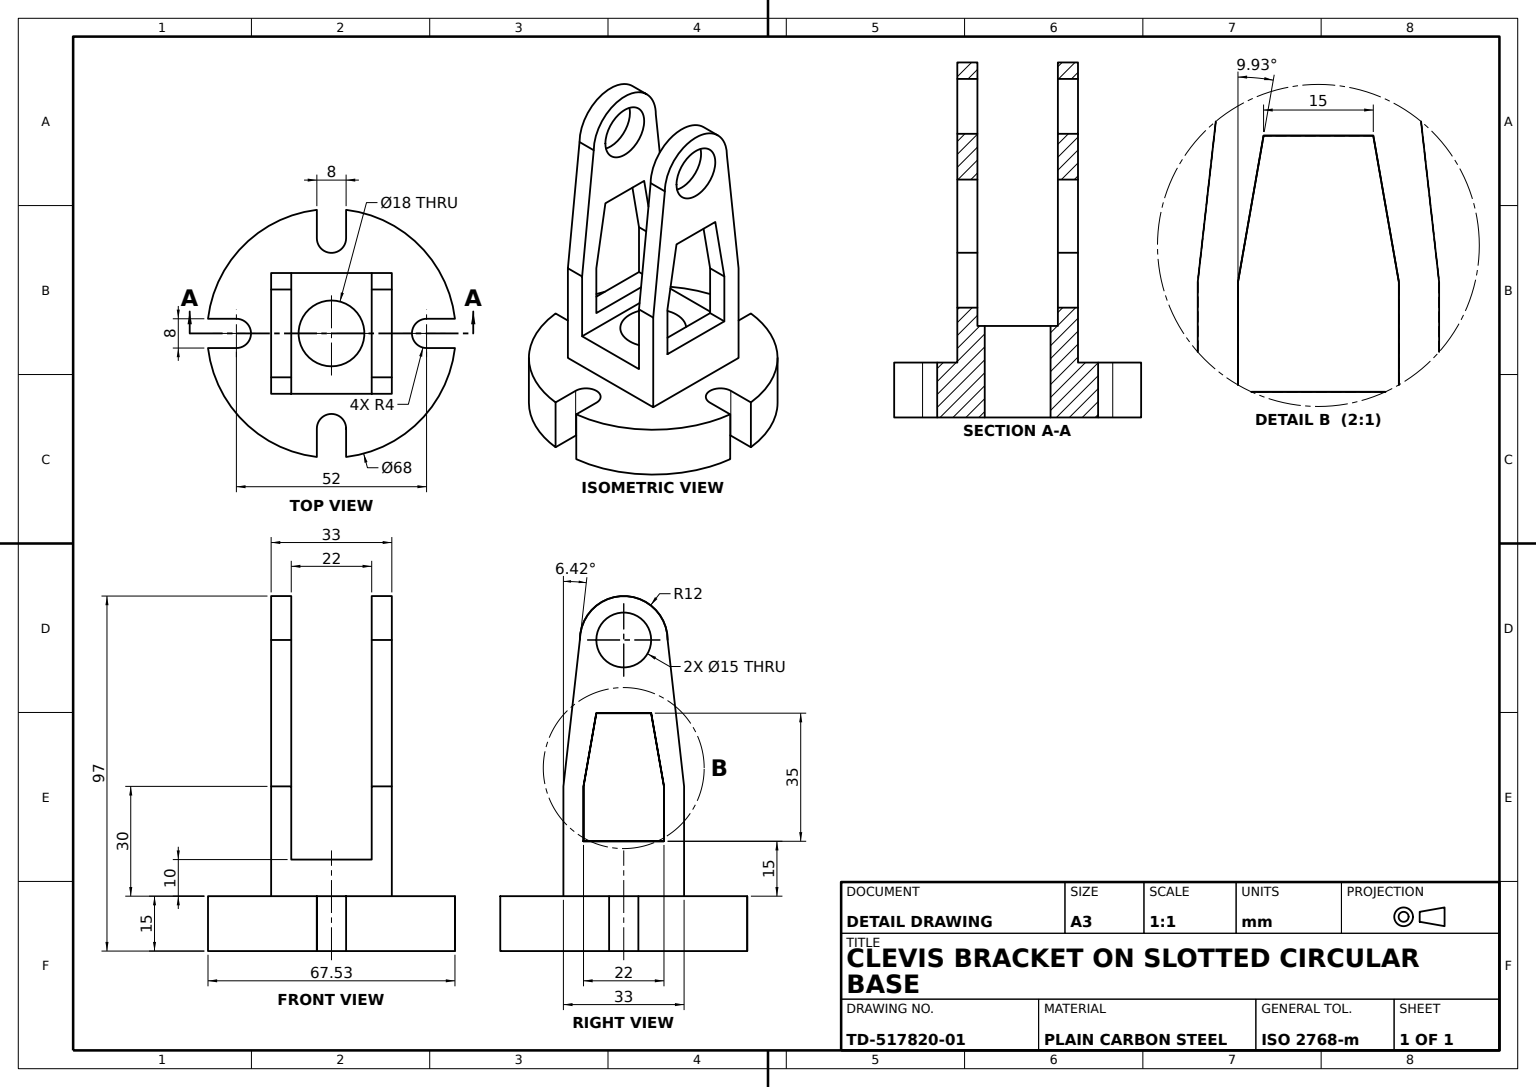
ISO-10303-21;
HEADER;
FILE_DESCRIPTION((''),'2;1');
FILE_NAME('','',(''),(''),'','','');
FILE_SCHEMA(('AUTOMOTIVE_DESIGN'));
ENDSEC;
DATA;
#1=APPLICATION_CONTEXT('');
#2=PRODUCT_CONTEXT('',#1,'mechanical');
#3=PRODUCT('','','',(#2));
#4=PRODUCT_DEFINITION_FORMATION('','',#3);
#5=PRODUCT_DEFINITION_CONTEXT('',#1,'design');
#6=PRODUCT_DEFINITION('','',#4,#5);
#7=PRODUCT_DEFINITION_SHAPE('','',#6);
#8=(LENGTH_UNIT()NAMED_UNIT(*)SI_UNIT(.MILLI.,.METRE.));
#9=(NAMED_UNIT(*)PLANE_ANGLE_UNIT()SI_UNIT($,.RADIAN.));
#10=(NAMED_UNIT(*)SI_UNIT($,.STERADIAN.)SOLID_ANGLE_UNIT());
#11=UNCERTAINTY_MEASURE_WITH_UNIT(LENGTH_MEASURE(1.E-05),#8,'distance_accuracy_value','');
#12=(GEOMETRIC_REPRESENTATION_CONTEXT(3)GLOBAL_UNCERTAINTY_ASSIGNED_CONTEXT((#11))GLOBAL_UNIT_ASSIGNED_CONTEXT((#8,#9,#10))REPRESENTATION_CONTEXT('',''));
#13=CARTESIAN_POINT('',(-33.763886,15.,-4.));
#14=VERTEX_POINT('',#13);
#15=CARTESIAN_POINT('',(-33.763886,0.,-4.));
#16=VERTEX_POINT('',#15);
#17=DIRECTION('',(0.,-1.,0.));
#18=VECTOR('',#17,1000.);
#19=LINE('',#13,#18);
#20=EDGE_CURVE('',#14,#16,#19,.T.);
#21=ORIENTED_EDGE('',*,*,#20,.F.);
#22=CARTESIAN_POINT('',(-4.,15.,-33.763886));
#23=VERTEX_POINT('',#22);
#24=CARTESIAN_POINT('',(0.,15.,0.));
#25=DIRECTION('',(0.,1.,0.));
#26=DIRECTION('',(0.,0.,1.));
#27=AXIS2_PLACEMENT_3D('',#24,#25,#26);
#28=CIRCLE('',#27,34.);
#29=EDGE_CURVE('',#23,#14,#28,.T.);
#30=ORIENTED_EDGE('',*,*,#29,.F.);
#31=CARTESIAN_POINT('',(-4.,0.,-33.763886));
#32=VERTEX_POINT('',#31);
#33=LINE('',#22,#18);
#34=EDGE_CURVE('',#23,#32,#33,.T.);
#35=ORIENTED_EDGE('',*,*,#34,.T.);
#36=CARTESIAN_POINT('',(0.,0.,0.));
#37=AXIS2_PLACEMENT_3D('',#36,#25,#26);
#38=CIRCLE('',#37,34.);
#39=EDGE_CURVE('',#32,#16,#38,.T.);
#40=ORIENTED_EDGE('',*,*,#39,.T.);
#41=EDGE_LOOP('',(#21,#30,#35,#40));
#42=FACE_OUTER_BOUND('',#41,.T.);
#43=DIRECTION('',(0.,0.,-1.));
#44=AXIS2_PLACEMENT_3D('',#24,#17,#43);
#45=CYLINDRICAL_SURFACE('',#44,34.);
#46=ADVANCED_FACE('',(#42),#45,.T.);
#47=CARTESIAN_POINT('',(11.,30.,11.));
#48=VERTEX_POINT('',#47);
#49=CARTESIAN_POINT('',(16.5,30.,11.));
#50=VERTEX_POINT('',#49);
#51=CARTESIAN_POINT('',(-37.5,30.,11.));
#52=DIRECTION('',(1.,0.,0.));
#53=VECTOR('',#52,1000.);
#54=LINE('',#51,#53);
#55=EDGE_CURVE('',#48,#50,#54,.T.);
#56=ORIENTED_EDGE('',*,*,#55,.T.);
#57=CARTESIAN_POINT('',(16.5,30.,-11.));
#58=VERTEX_POINT('',#57);
#59=CARTESIAN_POINT('',(16.5,30.,0.));
#60=VECTOR('',#43,1000.);
#61=LINE('',#59,#60);
#62=EDGE_CURVE('',#50,#58,#61,.T.);
#63=ORIENTED_EDGE('',*,*,#62,.T.);
#64=CARTESIAN_POINT('',(11.,30.,-11.));
#65=VERTEX_POINT('',#64);
#66=CARTESIAN_POINT('',(-37.5,30.,-11.));
#67=LINE('',#66,#53);
#68=EDGE_CURVE('',#65,#58,#67,.T.);
#69=ORIENTED_EDGE('',*,*,#68,.F.);
#70=CARTESIAN_POINT('',(11.,30.,0.));
#71=LINE('',#70,#60);
#72=EDGE_CURVE('',#48,#65,#71,.T.);
#73=ORIENTED_EDGE('',*,*,#72,.F.);
#74=EDGE_LOOP('',(#56,#63,#69,#73));
#75=FACE_OUTER_BOUND('',#74,.T.);
#76=CARTESIAN_POINT('',(-37.5,30.,0.));
#77=AXIS2_PLACEMENT_3D('',#76,#17,#43);
#78=PLANE('',#77);
#79=ADVANCED_FACE('',(#75),#78,.F.);
#80=CARTESIAN_POINT('',(4.,0.,26.));
#81=VERTEX_POINT('',#80);
#82=CARTESIAN_POINT('',(0.,0.,22.));
#83=VERTEX_POINT('',#82);
#84=CARTESIAN_POINT('',(0.,0.,26.));
#85=AXIS2_PLACEMENT_3D('',#84,#25,#26);
#86=CIRCLE('',#85,4.);
#87=EDGE_CURVE('',#81,#83,#86,.T.);
#88=ORIENTED_EDGE('',*,*,#87,.F.);
#89=CARTESIAN_POINT('',(4.,15.,26.));
#90=VERTEX_POINT('',#89);
#91=LINE('',#89,#18);
#92=EDGE_CURVE('',#90,#81,#91,.T.);
#93=ORIENTED_EDGE('',*,*,#92,.F.);
#94=CARTESIAN_POINT('',(0.,15.,22.));
#95=VERTEX_POINT('',#94);
#96=CARTESIAN_POINT('',(0.,15.,26.));
#97=AXIS2_PLACEMENT_3D('',#96,#25,#26);
#98=CIRCLE('',#97,4.);
#99=EDGE_CURVE('',#90,#95,#98,.T.);
#100=ORIENTED_EDGE('',*,*,#99,.T.);
#101=LINE('',#94,#18);
#102=EDGE_CURVE('',#95,#83,#101,.T.);
#103=ORIENTED_EDGE('',*,*,#102,.T.);
#104=EDGE_LOOP('',(#88,#93,#100,#103));
#105=FACE_OUTER_BOUND('',#104,.T.);
#106=AXIS2_PLACEMENT_3D('',#96,#17,#43);
#107=CYLINDRICAL_SURFACE('',#106,4.);
#108=ADVANCED_FACE('',(#105),#107,.F.);
#109=CARTESIAN_POINT('',(-11.,30.,11.));
#110=VERTEX_POINT('',#109);
#111=CARTESIAN_POINT('',(-11.,30.,-11.));
#112=VERTEX_POINT('',#111);
#113=CARTESIAN_POINT('',(-11.,30.,0.));
#114=LINE('',#113,#60);
#115=EDGE_CURVE('',#110,#112,#114,.T.);
#116=ORIENTED_EDGE('',*,*,#115,.T.);
#117=CARTESIAN_POINT('',(-16.5,30.,-11.));
#118=VERTEX_POINT('',#117);
#119=EDGE_CURVE('',#118,#112,#67,.T.);
#120=ORIENTED_EDGE('',*,*,#119,.F.);
#121=CARTESIAN_POINT('',(-16.5,30.,11.));
#122=VERTEX_POINT('',#121);
#123=CARTESIAN_POINT('',(-16.5,30.,0.));
#124=VECTOR('',#26,1000.);
#125=LINE('',#123,#124);
#126=EDGE_CURVE('',#118,#122,#125,.T.);
#127=ORIENTED_EDGE('',*,*,#126,.T.);
#128=EDGE_CURVE('',#122,#110,#54,.T.);
#129=ORIENTED_EDGE('',*,*,#128,.T.);
#130=EDGE_LOOP('',(#116,#120,#127,#129));
#131=FACE_OUTER_BOUND('',#130,.T.);
#132=ADVANCED_FACE('',(#131),#78,.F.);
#133=CARTESIAN_POINT('',(-16.5,15.,16.5));
#134=VERTEX_POINT('',#133);
#135=CARTESIAN_POINT('',(-16.5,15.,-16.5));
#136=VERTEX_POINT('',#135);
#137=CARTESIAN_POINT('',(-16.5,15.,0.));
#138=LINE('',#137,#60);
#139=EDGE_CURVE('',#134,#136,#138,.T.);
#140=ORIENTED_EDGE('',*,*,#139,.F.);
#141=CARTESIAN_POINT('',(-16.5,45.,16.5));
#142=VERTEX_POINT('',#141);
#143=CARTESIAN_POINT('',(-16.5,85.,16.5));
#144=LINE('',#143,#18);
#145=EDGE_CURVE('',#142,#134,#144,.T.);
#146=ORIENTED_EDGE('',*,*,#145,.F.);
#147=CARTESIAN_POINT('',(-16.5,85.,12.));
#148=VERTEX_POINT('',#147);
#149=CARTESIAN_POINT('',(-16.5,86.333128,11.850023));
#150=DIRECTION('',(0.,0.993731316,-0.111794773));
#151=VECTOR('',#150,1000.);
#152=LINE('',#149,#151);
#153=EDGE_CURVE('',#142,#148,#152,.T.);
#154=ORIENTED_EDGE('',*,*,#153,.T.);
#155=CARTESIAN_POINT('',(-16.5,85.,-12.));
#156=VERTEX_POINT('',#155);
#157=CARTESIAN_POINT('',(-16.5,85.,0.));
#158=DIRECTION('',(-1.,0.,0.));
#159=AXIS2_PLACEMENT_3D('',#157,#158,#26);
#160=CIRCLE('',#159,12.);
#161=EDGE_CURVE('',#148,#156,#160,.T.);
#162=ORIENTED_EDGE('',*,*,#161,.T.);
#163=CARTESIAN_POINT('',(-16.5,45.,-16.5));
#164=VERTEX_POINT('',#163);
#165=CARTESIAN_POINT('',(-16.5,86.333128,-11.850023));
#166=DIRECTION('',(0.,0.993731316,0.111794773));
#167=VECTOR('',#166,1000.);
#168=LINE('',#165,#167);
#169=EDGE_CURVE('',#164,#156,#168,.T.);
#170=ORIENTED_EDGE('',*,*,#169,.F.);
#171=CARTESIAN_POINT('',(-16.5,85.,-16.5));
#172=LINE('',#171,#18);
#173=EDGE_CURVE('',#164,#136,#172,.T.);
#174=ORIENTED_EDGE('',*,*,#173,.T.);
#175=EDGE_LOOP('',(#140,#146,#154,#162,#170,#174));
#176=FACE_OUTER_BOUND('',#175,.T.);
#177=CARTESIAN_POINT('',(-16.5,85.,-7.5));
#178=VERTEX_POINT('',#177);
#179=CARTESIAN_POINT('',(-16.5,85.,7.5));
#180=VERTEX_POINT('',#179);
#181=CIRCLE('',#159,7.5);
#182=EDGE_CURVE('',#178,#180,#181,.T.);
#183=ORIENTED_EDGE('',*,*,#182,.F.);
#184=EDGE_CURVE('',#180,#178,#181,.T.);
#185=ORIENTED_EDGE('',*,*,#184,.F.);
#186=EDGE_LOOP('',(#183,#185));
#187=FACE_BOUND('',#186,.T.);
#188=CARTESIAN_POINT('',(-16.5,45.,11.));
#189=VERTEX_POINT('',#188);
#190=CARTESIAN_POINT('',(-16.5,85.,11.));
#191=LINE('',#190,#18);
#192=EDGE_CURVE('',#189,#122,#191,.T.);
#193=ORIENTED_EDGE('',*,*,#192,.T.);
#194=ORIENTED_EDGE('',*,*,#126,.F.);
#195=CARTESIAN_POINT('',(-16.5,45.,-11.));
#196=VERTEX_POINT('',#195);
#197=CARTESIAN_POINT('',(-16.5,85.,-11.));
#198=LINE('',#197,#18);
#199=EDGE_CURVE('',#196,#118,#198,.T.);
#200=ORIENTED_EDGE('',*,*,#199,.F.);
#201=CARTESIAN_POINT('',(-16.5,65.,-7.5));
#202=VERTEX_POINT('',#201);
#203=CARTESIAN_POINT('',(-16.5,85.6792,-3.88114));
#204=DIRECTION('',(0.,0.985030467,0.172380332));
#205=VECTOR('',#204,1000.);
#206=LINE('',#203,#205);
#207=EDGE_CURVE('',#196,#202,#206,.T.);
#208=ORIENTED_EDGE('',*,*,#207,.T.);
#209=CARTESIAN_POINT('',(-16.5,65.,7.5));
#210=VERTEX_POINT('',#209);
#211=CARTESIAN_POINT('',(-16.5,65.,0.));
#212=LINE('',#211,#124);
#213=EDGE_CURVE('',#202,#210,#212,.T.);
#214=ORIENTED_EDGE('',*,*,#213,.T.);
#215=CARTESIAN_POINT('',(-16.5,85.6792,3.88114));
#216=DIRECTION('',(0.,0.985030467,-0.172380332));
#217=VECTOR('',#216,1000.);
#218=LINE('',#215,#217);
#219=EDGE_CURVE('',#189,#210,#218,.T.);
#220=ORIENTED_EDGE('',*,*,#219,.F.);
#221=EDGE_LOOP('',(#193,#194,#200,#208,#214,#220));
#222=FACE_BOUND('',#221,.T.);
#223=PLANE('',#159);
#224=ADVANCED_FACE('',(#176,#187,#222),#223,.T.);
#225=CARTESIAN_POINT('',(11.,85.,7.5));
#226=VERTEX_POINT('',#225);
#227=CARTESIAN_POINT('',(16.5,85.,7.5));
#228=VERTEX_POINT('',#227);
#229=CARTESIAN_POINT('',(-37.5,85.,7.5));
#230=LINE('',#229,#53);
#231=EDGE_CURVE('',#226,#228,#230,.T.);
#232=ORIENTED_EDGE('',*,*,#231,.T.);
#233=CARTESIAN_POINT('',(16.5,85.,-7.5));
#234=VERTEX_POINT('',#233);
#235=CARTESIAN_POINT('',(16.5,85.,0.));
#236=AXIS2_PLACEMENT_3D('',#235,#52,#43);
#237=CIRCLE('',#236,7.5);
#238=EDGE_CURVE('',#228,#234,#237,.T.);
#239=ORIENTED_EDGE('',*,*,#238,.T.);
#240=CARTESIAN_POINT('',(11.,85.,-7.5));
#241=VERTEX_POINT('',#240);
#242=CARTESIAN_POINT('',(-37.5,85.,-7.5));
#243=LINE('',#242,#53);
#244=EDGE_CURVE('',#241,#234,#243,.T.);
#245=ORIENTED_EDGE('',*,*,#244,.F.);
#246=CARTESIAN_POINT('',(11.,85.,0.));
#247=AXIS2_PLACEMENT_3D('',#246,#52,#43);
#248=CIRCLE('',#247,7.5);
#249=EDGE_CURVE('',#226,#241,#248,.T.);
#250=ORIENTED_EDGE('',*,*,#249,.F.);
#251=EDGE_LOOP('',(#232,#239,#245,#250));
#252=FACE_OUTER_BOUND('',#251,.T.);
#253=CARTESIAN_POINT('',(-37.5,85.,0.));
#254=AXIS2_PLACEMENT_3D('',#253,#52,#43);
#255=CYLINDRICAL_SURFACE('',#254,7.5);
#256=ADVANCED_FACE('',(#252),#255,.F.);
#257=CARTESIAN_POINT('',(11.,65.,7.5));
#258=VERTEX_POINT('',#257);
#259=CARTESIAN_POINT('',(11.,45.,11.));
#260=VERTEX_POINT('',#259);
#261=CARTESIAN_POINT('',(11.,85.6792,3.88114));
#262=DIRECTION('',(0.,-0.985030467,0.172380332));
#263=VECTOR('',#262,1000.);
#264=LINE('',#261,#263);
#265=EDGE_CURVE('',#258,#260,#264,.T.);
#266=ORIENTED_EDGE('',*,*,#265,.F.);
#267=CARTESIAN_POINT('',(16.5,65.,7.5));
#268=VERTEX_POINT('',#267);
#269=CARTESIAN_POINT('',(-37.5,65.,7.5));
#270=LINE('',#269,#53);
#271=EDGE_CURVE('',#258,#268,#270,.T.);
#272=ORIENTED_EDGE('',*,*,#271,.T.);
#273=CARTESIAN_POINT('',(16.5,45.,11.));
#274=VERTEX_POINT('',#273);
#275=CARTESIAN_POINT('',(16.5,3.204973,18.31413));
#276=LINE('',#275,#263);
#277=EDGE_CURVE('',#268,#274,#276,.T.);
#278=ORIENTED_EDGE('',*,*,#277,.T.);
#279=CARTESIAN_POINT('',(-37.5,45.,11.));
#280=LINE('',#279,#53);
#281=EDGE_CURVE('',#260,#274,#280,.T.);
#282=ORIENTED_EDGE('',*,*,#281,.F.);
#283=EDGE_LOOP('',(#266,#272,#278,#282));
#284=FACE_OUTER_BOUND('',#283,.T.);
#285=CARTESIAN_POINT('',(-37.5,3.204973,18.31413));
#286=DIRECTION('',(0.,0.172380332,0.985030467));
#287=AXIS2_PLACEMENT_3D('',#285,#286,#262);
#288=PLANE('',#287);
#289=ADVANCED_FACE('',(#284),#288,.F.);
#290=CARTESIAN_POINT('',(-11.,85.,-12.));
#291=VERTEX_POINT('',#290);
#292=CARTESIAN_POINT('',(-11.,45.,-16.5));
#293=VERTEX_POINT('',#292);
#294=CARTESIAN_POINT('',(-11.,86.333128,-11.850023));
#295=DIRECTION('',(0.,-0.993731316,-0.111794773));
#296=VECTOR('',#295,1000.);
#297=LINE('',#294,#296);
#298=EDGE_CURVE('',#291,#293,#297,.T.);
#299=ORIENTED_EDGE('',*,*,#298,.T.);
#300=CARTESIAN_POINT('',(-37.5,45.,-16.5));
#301=LINE('',#300,#53);
#302=EDGE_CURVE('',#164,#293,#301,.T.);
#303=ORIENTED_EDGE('',*,*,#302,.F.);
#304=ORIENTED_EDGE('',*,*,#169,.T.);
#305=CARTESIAN_POINT('',(0.,85.,-12.));
#306=LINE('',#305,#53);
#307=EDGE_CURVE('',#156,#291,#306,.T.);
#308=ORIENTED_EDGE('',*,*,#307,.T.);
#309=EDGE_LOOP('',(#299,#303,#304,#308));
#310=FACE_OUTER_BOUND('',#309,.T.);
#311=CARTESIAN_POINT('',(-37.5,2.395464,-21.29301));
#312=DIRECTION('',(0.,-0.111794773,0.993731316));
#313=AXIS2_PLACEMENT_3D('',#311,#312,#295);
#314=PLANE('',#313);
#315=ADVANCED_FACE('',(#310),#314,.F.);
#316=CARTESIAN_POINT('',(33.763886,15.,-4.));
#317=VERTEX_POINT('',#316);
#318=CARTESIAN_POINT('',(33.763886,0.,-4.));
#319=VERTEX_POINT('',#318);
#320=LINE('',#316,#18);
#321=EDGE_CURVE('',#317,#319,#320,.T.);
#322=ORIENTED_EDGE('',*,*,#321,.T.);
#323=CARTESIAN_POINT('',(4.,0.,-33.763886));
#324=VERTEX_POINT('',#323);
#325=EDGE_CURVE('',#319,#324,#38,.T.);
#326=ORIENTED_EDGE('',*,*,#325,.T.);
#327=CARTESIAN_POINT('',(4.,15.,-33.763886));
#328=VERTEX_POINT('',#327);
#329=LINE('',#327,#18);
#330=EDGE_CURVE('',#328,#324,#329,.T.);
#331=ORIENTED_EDGE('',*,*,#330,.F.);
#332=EDGE_CURVE('',#317,#328,#28,.T.);
#333=ORIENTED_EDGE('',*,*,#332,.F.);
#334=EDGE_LOOP('',(#322,#326,#331,#333));
#335=FACE_OUTER_BOUND('',#334,.T.);
#336=ADVANCED_FACE('',(#335),#45,.T.);
#337=CARTESIAN_POINT('',(0.,25.,-9.));
#338=VERTEX_POINT('',#337);
#339=CARTESIAN_POINT('',(0.,25.,9.));
#340=VERTEX_POINT('',#339);
#341=CARTESIAN_POINT('',(0.,25.,0.));
#342=AXIS2_PLACEMENT_3D('',#341,#17,#26);
#343=CIRCLE('',#342,9.);
#344=EDGE_CURVE('',#338,#340,#343,.T.);
#345=ORIENTED_EDGE('',*,*,#344,.T.);
#346=EDGE_CURVE('',#340,#338,#343,.T.);
#347=ORIENTED_EDGE('',*,*,#346,.T.);
#348=EDGE_LOOP('',(#345,#347));
#349=FACE_BOUND('',#348,.T.);
#350=CARTESIAN_POINT('',(11.,25.,-16.5));
#351=VERTEX_POINT('',#350);
#352=CARTESIAN_POINT('',(11.,25.,16.5));
#353=VERTEX_POINT('',#352);
#354=CARTESIAN_POINT('',(11.,25.,0.));
#355=LINE('',#354,#124);
#356=EDGE_CURVE('',#351,#353,#355,.T.);
#357=ORIENTED_EDGE('',*,*,#356,.F.);
#358=CARTESIAN_POINT('',(-11.,25.,-16.5));
#359=VERTEX_POINT('',#358);
#360=CARTESIAN_POINT('',(0.,25.,-16.5));
#361=LINE('',#360,#53);
#362=EDGE_CURVE('',#359,#351,#361,.T.);
#363=ORIENTED_EDGE('',*,*,#362,.F.);
#364=CARTESIAN_POINT('',(-11.,25.,16.5));
#365=VERTEX_POINT('',#364);
#366=CARTESIAN_POINT('',(-11.,25.,0.));
#367=LINE('',#366,#124);
#368=EDGE_CURVE('',#359,#365,#367,.T.);
#369=ORIENTED_EDGE('',*,*,#368,.T.);
#370=CARTESIAN_POINT('',(0.,25.,16.5));
#371=LINE('',#370,#53);
#372=EDGE_CURVE('',#365,#353,#371,.T.);
#373=ORIENTED_EDGE('',*,*,#372,.T.);
#374=EDGE_LOOP('',(#357,#363,#369,#373));
#375=FACE_OUTER_BOUND('',#374,.T.);
#376=AXIS2_PLACEMENT_3D('',#341,#25,#26);
#377=PLANE('',#376);
#378=ADVANCED_FACE('',(#349,#375),#377,.T.);
#379=CARTESIAN_POINT('',(-4.,15.,26.));
#380=VERTEX_POINT('',#379);
#381=CARTESIAN_POINT('',(-4.,0.,26.));
#382=VERTEX_POINT('',#381);
#383=LINE('',#379,#18);
#384=EDGE_CURVE('',#380,#382,#383,.T.);
#385=ORIENTED_EDGE('',*,*,#384,.T.);
#386=EDGE_CURVE('',#83,#382,#86,.T.);
#387=ORIENTED_EDGE('',*,*,#386,.F.);
#388=ORIENTED_EDGE('',*,*,#102,.F.);
#389=EDGE_CURVE('',#95,#380,#98,.T.);
#390=ORIENTED_EDGE('',*,*,#389,.T.);
#391=EDGE_LOOP('',(#385,#387,#388,#390));
#392=FACE_OUTER_BOUND('',#391,.T.);
#393=ADVANCED_FACE('',(#392),#107,.F.);
#394=CARTESIAN_POINT('',(-33.763886,15.,4.));
#395=VERTEX_POINT('',#394);
#396=CARTESIAN_POINT('',(-4.,15.,33.763886));
#397=VERTEX_POINT('',#396);
#398=EDGE_CURVE('',#395,#397,#28,.T.);
#399=ORIENTED_EDGE('',*,*,#398,.F.);
#400=CARTESIAN_POINT('',(-33.763886,0.,4.));
#401=VERTEX_POINT('',#400);
#402=LINE('',#394,#18);
#403=EDGE_CURVE('',#395,#401,#402,.T.);
#404=ORIENTED_EDGE('',*,*,#403,.T.);
#405=CARTESIAN_POINT('',(-4.,0.,33.763886));
#406=VERTEX_POINT('',#405);
#407=EDGE_CURVE('',#401,#406,#38,.T.);
#408=ORIENTED_EDGE('',*,*,#407,.T.);
#409=LINE('',#396,#18);
#410=EDGE_CURVE('',#397,#406,#409,.T.);
#411=ORIENTED_EDGE('',*,*,#410,.F.);
#412=EDGE_LOOP('',(#399,#404,#408,#411));
#413=FACE_OUTER_BOUND('',#412,.T.);
#414=ADVANCED_FACE('',(#413),#45,.T.);
#415=CARTESIAN_POINT('',(-11.,65.,7.5));
#416=VERTEX_POINT('',#415);
#417=EDGE_CURVE('',#210,#416,#270,.T.);
#418=ORIENTED_EDGE('',*,*,#417,.T.);
#419=CARTESIAN_POINT('',(-11.,45.,11.));
#420=VERTEX_POINT('',#419);
#421=CARTESIAN_POINT('',(-11.,85.6792,3.88114));
#422=LINE('',#421,#263);
#423=EDGE_CURVE('',#416,#420,#422,.T.);
#424=ORIENTED_EDGE('',*,*,#423,.T.);
#425=EDGE_CURVE('',#189,#420,#280,.T.);
#426=ORIENTED_EDGE('',*,*,#425,.F.);
#427=ORIENTED_EDGE('',*,*,#219,.T.);
#428=EDGE_LOOP('',(#418,#424,#426,#427));
#429=FACE_OUTER_BOUND('',#428,.T.);
#430=ADVANCED_FACE('',(#429),#288,.F.);
#431=CARTESIAN_POINT('',(11.,85.,-12.));
#432=VERTEX_POINT('',#431);
#433=CARTESIAN_POINT('',(11.,45.,-16.5));
#434=VERTEX_POINT('',#433);
#435=CARTESIAN_POINT('',(11.,86.333128,-11.850023));
#436=LINE('',#435,#296);
#437=EDGE_CURVE('',#432,#434,#436,.T.);
#438=ORIENTED_EDGE('',*,*,#437,.F.);
#439=CARTESIAN_POINT('',(16.5,85.,-12.));
#440=VERTEX_POINT('',#439);
#441=CARTESIAN_POINT('',(-37.5,85.,-12.));
#442=LINE('',#441,#53);
#443=EDGE_CURVE('',#432,#440,#442,.T.);
#444=ORIENTED_EDGE('',*,*,#443,.T.);
#445=CARTESIAN_POINT('',(16.5,45.,-16.5));
#446=VERTEX_POINT('',#445);
#447=CARTESIAN_POINT('',(16.5,2.395464,-21.29301));
#448=LINE('',#447,#296);
#449=EDGE_CURVE('',#440,#446,#448,.T.);
#450=ORIENTED_EDGE('',*,*,#449,.T.);
#451=EDGE_CURVE('',#434,#446,#301,.T.);
#452=ORIENTED_EDGE('',*,*,#451,.F.);
#453=EDGE_LOOP('',(#438,#444,#450,#452));
#454=FACE_OUTER_BOUND('',#453,.T.);
#455=ADVANCED_FACE('',(#454),#314,.F.);
#456=CARTESIAN_POINT('',(33.763886,15.,4.));
#457=VERTEX_POINT('',#456);
#458=CARTESIAN_POINT('',(33.763886,0.,4.));
#459=VERTEX_POINT('',#458);
#460=LINE('',#456,#18);
#461=EDGE_CURVE('',#457,#459,#460,.T.);
#462=ORIENTED_EDGE('',*,*,#461,.F.);
#463=CARTESIAN_POINT('',(4.,15.,33.763886));
#464=VERTEX_POINT('',#463);
#465=EDGE_CURVE('',#464,#457,#28,.T.);
#466=ORIENTED_EDGE('',*,*,#465,.F.);
#467=CARTESIAN_POINT('',(4.,0.,33.763886));
#468=VERTEX_POINT('',#467);
#469=LINE('',#463,#18);
#470=EDGE_CURVE('',#464,#468,#469,.T.);
#471=ORIENTED_EDGE('',*,*,#470,.T.);
#472=EDGE_CURVE('',#468,#459,#38,.T.);
#473=ORIENTED_EDGE('',*,*,#472,.T.);
#474=EDGE_LOOP('',(#462,#466,#471,#473));
#475=FACE_OUTER_BOUND('',#474,.T.);
#476=ADVANCED_FACE('',(#475),#45,.T.);
#477=ORIENTED_EDGE('',*,*,#470,.F.);
#478=CARTESIAN_POINT('',(4.,15.,0.));
#479=LINE('',#478,#124);
#480=EDGE_CURVE('',#90,#464,#479,.T.);
#481=ORIENTED_EDGE('',*,*,#480,.F.);
#482=ORIENTED_EDGE('',*,*,#92,.T.);
#483=CARTESIAN_POINT('',(4.,0.,0.));
#484=LINE('',#483,#124);
#485=EDGE_CURVE('',#81,#468,#484,.T.);
#486=ORIENTED_EDGE('',*,*,#485,.T.);
#487=EDGE_LOOP('',(#477,#481,#482,#486));
#488=FACE_OUTER_BOUND('',#487,.T.);
#489=AXIS2_PLACEMENT_3D('',#478,#52,#43);
#490=PLANE('',#489);
#491=ADVANCED_FACE('',(#488),#490,.F.);
#492=CARTESIAN_POINT('',(16.5,65.,-7.5));
#493=VERTEX_POINT('',#492);
#494=CARTESIAN_POINT('',(16.5,65.,0.));
#495=LINE('',#494,#60);
#496=EDGE_CURVE('',#268,#493,#495,.T.);
#497=ORIENTED_EDGE('',*,*,#496,.F.);
#498=ORIENTED_EDGE('',*,*,#271,.F.);
#499=CARTESIAN_POINT('',(11.,65.,-7.5));
#500=VERTEX_POINT('',#499);
#501=CARTESIAN_POINT('',(11.,65.,0.));
#502=LINE('',#501,#60);
#503=EDGE_CURVE('',#258,#500,#502,.T.);
#504=ORIENTED_EDGE('',*,*,#503,.T.);
#505=CARTESIAN_POINT('',(-37.5,65.,-7.5));
#506=LINE('',#505,#53);
#507=EDGE_CURVE('',#500,#493,#506,.T.);
#508=ORIENTED_EDGE('',*,*,#507,.T.);
#509=EDGE_LOOP('',(#497,#498,#504,#508));
#510=FACE_OUTER_BOUND('',#509,.T.);
#511=CARTESIAN_POINT('',(-37.5,65.,0.));
#512=AXIS2_PLACEMENT_3D('',#511,#17,#43);
#513=PLANE('',#512);
#514=ADVANCED_FACE('',(#510),#513,.T.);
#515=CARTESIAN_POINT('',(11.,45.,-11.));
#516=VERTEX_POINT('',#515);
#517=CARTESIAN_POINT('',(11.,85.6792,-3.88114));
#518=DIRECTION('',(0.,-0.985030467,-0.172380332));
#519=VECTOR('',#518,1000.);
#520=LINE('',#517,#519);
#521=EDGE_CURVE('',#500,#516,#520,.T.);
#522=ORIENTED_EDGE('',*,*,#521,.T.);
#523=CARTESIAN_POINT('',(16.5,45.,-11.));
#524=VERTEX_POINT('',#523);
#525=CARTESIAN_POINT('',(-37.5,45.,-11.));
#526=LINE('',#525,#53);
#527=EDGE_CURVE('',#516,#524,#526,.T.);
#528=ORIENTED_EDGE('',*,*,#527,.T.);
#529=CARTESIAN_POINT('',(16.5,3.204973,-18.31413));
#530=LINE('',#529,#519);
#531=EDGE_CURVE('',#493,#524,#530,.T.);
#532=ORIENTED_EDGE('',*,*,#531,.F.);
#533=ORIENTED_EDGE('',*,*,#507,.F.);
#534=EDGE_LOOP('',(#522,#528,#532,#533));
#535=FACE_OUTER_BOUND('',#534,.T.);
#536=CARTESIAN_POINT('',(-37.5,3.204973,-18.31413));
#537=DIRECTION('',(0.,-0.172380332,0.985030467));
#538=AXIS2_PLACEMENT_3D('',#536,#537,#518);
#539=PLANE('',#538);
#540=ADVANCED_FACE('',(#535),#539,.T.);
#541=EDGE_CURVE('',#234,#228,#237,.T.);
#542=ORIENTED_EDGE('',*,*,#541,.T.);
#543=ORIENTED_EDGE('',*,*,#231,.F.);
#544=EDGE_CURVE('',#241,#226,#248,.T.);
#545=ORIENTED_EDGE('',*,*,#544,.F.);
#546=ORIENTED_EDGE('',*,*,#244,.T.);
#547=EDGE_LOOP('',(#542,#543,#545,#546));
#548=FACE_OUTER_BOUND('',#547,.T.);
#549=ADVANCED_FACE('',(#548),#255,.F.);
#550=CARTESIAN_POINT('',(-4.,15.,-26.));
#551=VERTEX_POINT('',#550);
#552=CARTESIAN_POINT('',(-4.,0.,-26.));
#553=VERTEX_POINT('',#552);
#554=LINE('',#550,#18);
#555=EDGE_CURVE('',#551,#553,#554,.T.);
#556=ORIENTED_EDGE('',*,*,#555,.T.);
#557=CARTESIAN_POINT('',(-4.,0.,0.));
#558=LINE('',#557,#60);
#559=EDGE_CURVE('',#553,#32,#558,.T.);
#560=ORIENTED_EDGE('',*,*,#559,.T.);
#561=ORIENTED_EDGE('',*,*,#34,.F.);
#562=CARTESIAN_POINT('',(-4.,15.,0.));
#563=LINE('',#562,#60);
#564=EDGE_CURVE('',#551,#23,#563,.T.);
#565=ORIENTED_EDGE('',*,*,#564,.F.);
#566=EDGE_LOOP('',(#556,#560,#561,#565));
#567=FACE_OUTER_BOUND('',#566,.T.);
#568=AXIS2_PLACEMENT_3D('',#562,#158,#26);
#569=PLANE('',#568);
#570=ADVANCED_FACE('',(#567),#569,.F.);
#571=CARTESIAN_POINT('',(11.,45.,16.5));
#572=VERTEX_POINT('',#571);
#573=CARTESIAN_POINT('',(16.5,45.,16.5));
#574=VERTEX_POINT('',#573);
#575=CARTESIAN_POINT('',(-37.5,45.,16.5));
#576=LINE('',#575,#53);
#577=EDGE_CURVE('',#572,#574,#576,.T.);
#578=ORIENTED_EDGE('',*,*,#577,.T.);
#579=CARTESIAN_POINT('',(16.5,85.,12.));
#580=VERTEX_POINT('',#579);
#581=CARTESIAN_POINT('',(16.5,2.395464,21.29301));
#582=DIRECTION('',(0.,-0.993731316,0.111794773));
#583=VECTOR('',#582,1000.);
#584=LINE('',#581,#583);
#585=EDGE_CURVE('',#580,#574,#584,.T.);
#586=ORIENTED_EDGE('',*,*,#585,.F.);
#587=CARTESIAN_POINT('',(11.,85.,12.));
#588=VERTEX_POINT('',#587);
#589=CARTESIAN_POINT('',(-37.5,85.,12.));
#590=LINE('',#589,#53);
#591=EDGE_CURVE('',#588,#580,#590,.T.);
#592=ORIENTED_EDGE('',*,*,#591,.F.);
#593=CARTESIAN_POINT('',(11.,86.333128,11.850023));
#594=LINE('',#593,#583);
#595=EDGE_CURVE('',#588,#572,#594,.T.);
#596=ORIENTED_EDGE('',*,*,#595,.T.);
#597=EDGE_LOOP('',(#578,#586,#592,#596));
#598=FACE_OUTER_BOUND('',#597,.T.);
#599=CARTESIAN_POINT('',(-37.5,2.395464,21.29301));
#600=DIRECTION('',(0.,0.111794773,0.993731316));
#601=AXIS2_PLACEMENT_3D('',#599,#600,#582);
#602=PLANE('',#601);
#603=ADVANCED_FACE('',(#598),#602,.T.);
#604=CARTESIAN_POINT('',(-11.,85.,12.));
#605=VERTEX_POINT('',#604);
#606=CARTESIAN_POINT('',(0.,85.,12.));
#607=LINE('',#606,#53);
#608=EDGE_CURVE('',#148,#605,#607,.T.);
#609=ORIENTED_EDGE('',*,*,#608,.F.);
#610=ORIENTED_EDGE('',*,*,#153,.F.);
#611=CARTESIAN_POINT('',(-11.,45.,16.5));
#612=VERTEX_POINT('',#611);
#613=EDGE_CURVE('',#142,#612,#576,.T.);
#614=ORIENTED_EDGE('',*,*,#613,.T.);
#615=CARTESIAN_POINT('',(-11.,86.333128,11.850023));
#616=LINE('',#615,#583);
#617=EDGE_CURVE('',#605,#612,#616,.T.);
#618=ORIENTED_EDGE('',*,*,#617,.F.);
#619=EDGE_LOOP('',(#609,#610,#614,#618));
#620=FACE_OUTER_BOUND('',#619,.T.);
#621=ADVANCED_FACE('',(#620),#602,.T.);
#622=CARTESIAN_POINT('',(-11.,65.,-7.5));
#623=VERTEX_POINT('',#622);
#624=EDGE_CURVE('',#202,#623,#506,.T.);
#625=ORIENTED_EDGE('',*,*,#624,.T.);
#626=CARTESIAN_POINT('',(-11.,65.,0.));
#627=LINE('',#626,#60);
#628=EDGE_CURVE('',#416,#623,#627,.T.);
#629=ORIENTED_EDGE('',*,*,#628,.F.);
#630=ORIENTED_EDGE('',*,*,#417,.F.);
#631=ORIENTED_EDGE('',*,*,#213,.F.);
#632=EDGE_LOOP('',(#625,#629,#630,#631));
#633=FACE_OUTER_BOUND('',#632,.T.);
#634=ADVANCED_FACE('',(#633),#513,.T.);
#635=CARTESIAN_POINT('',(16.5,15.,16.5));
#636=VERTEX_POINT('',#635);
#637=CARTESIAN_POINT('',(16.5,85.,16.5));
#638=LINE('',#637,#18);
#639=EDGE_CURVE('',#574,#636,#638,.T.);
#640=ORIENTED_EDGE('',*,*,#639,.T.);
#641=CARTESIAN_POINT('',(16.5,15.,-16.5));
#642=VERTEX_POINT('',#641);
#643=CARTESIAN_POINT('',(16.5,15.,0.));
#644=LINE('',#643,#60);
#645=EDGE_CURVE('',#636,#642,#644,.T.);
#646=ORIENTED_EDGE('',*,*,#645,.T.);
#647=CARTESIAN_POINT('',(16.5,85.,-16.5));
#648=LINE('',#647,#18);
#649=EDGE_CURVE('',#446,#642,#648,.T.);
#650=ORIENTED_EDGE('',*,*,#649,.F.);
#651=ORIENTED_EDGE('',*,*,#449,.F.);
#652=CIRCLE('',#236,12.);
#653=EDGE_CURVE('',#440,#580,#652,.T.);
#654=ORIENTED_EDGE('',*,*,#653,.T.);
#655=ORIENTED_EDGE('',*,*,#585,.T.);
#656=EDGE_LOOP('',(#640,#646,#650,#651,#654,#655));
#657=FACE_OUTER_BOUND('',#656,.T.);
#658=CARTESIAN_POINT('',(16.5,0.,11.));
#659=VECTOR('',#25,1000.);
#660=LINE('',#658,#659);
#661=EDGE_CURVE('',#50,#274,#660,.T.);
#662=ORIENTED_EDGE('',*,*,#661,.T.);
#663=ORIENTED_EDGE('',*,*,#277,.F.);
#664=ORIENTED_EDGE('',*,*,#496,.T.);
#665=ORIENTED_EDGE('',*,*,#531,.T.);
#666=CARTESIAN_POINT('',(16.5,0.,-11.));
#667=LINE('',#666,#659);
#668=EDGE_CURVE('',#58,#524,#667,.T.);
#669=ORIENTED_EDGE('',*,*,#668,.F.);
#670=ORIENTED_EDGE('',*,*,#62,.F.);
#671=EDGE_LOOP('',(#662,#663,#664,#665,#669,#670));
#672=FACE_BOUND('',#671,.T.);
#673=ORIENTED_EDGE('',*,*,#238,.F.);
#674=ORIENTED_EDGE('',*,*,#541,.F.);
#675=EDGE_LOOP('',(#673,#674));
#676=FACE_BOUND('',#675,.T.);
#677=AXIS2_PLACEMENT_3D('',#235,#158,#26);
#678=PLANE('',#677);
#679=ADVANCED_FACE('',(#657,#672,#676),#678,.F.);
#680=ORIENTED_EDGE('',*,*,#20,.T.);
#681=CARTESIAN_POINT('',(-26.,0.,-4.));
#682=VERTEX_POINT('',#681);
#683=CARTESIAN_POINT('',(0.,0.,-4.));
#684=VECTOR('',#158,1000.);
#685=LINE('',#683,#684);
#686=EDGE_CURVE('',#682,#16,#685,.T.);
#687=ORIENTED_EDGE('',*,*,#686,.F.);
#688=CARTESIAN_POINT('',(-26.,15.,-4.));
#689=VERTEX_POINT('',#688);
#690=LINE('',#688,#18);
#691=EDGE_CURVE('',#689,#682,#690,.T.);
#692=ORIENTED_EDGE('',*,*,#691,.F.);
#693=CARTESIAN_POINT('',(0.,15.,-4.));
#694=LINE('',#693,#684);
#695=EDGE_CURVE('',#689,#14,#694,.T.);
#696=ORIENTED_EDGE('',*,*,#695,.T.);
#697=EDGE_LOOP('',(#680,#687,#692,#696));
#698=FACE_OUTER_BOUND('',#697,.T.);
#699=AXIS2_PLACEMENT_3D('',#693,#26,#52);
#700=PLANE('',#699);
#701=ADVANCED_FACE('',(#698),#700,.T.);
#702=ORIENTED_EDGE('',*,*,#281,.T.);
#703=ORIENTED_EDGE('',*,*,#661,.F.);
#704=ORIENTED_EDGE('',*,*,#55,.F.);
#705=CARTESIAN_POINT('',(11.,85.,11.));
#706=LINE('',#705,#659);
#707=EDGE_CURVE('',#48,#260,#706,.T.);
#708=ORIENTED_EDGE('',*,*,#707,.T.);
#709=EDGE_LOOP('',(#702,#703,#704,#708));
#710=FACE_OUTER_BOUND('',#709,.T.);
#711=CARTESIAN_POINT('',(-37.5,0.,11.));
#712=AXIS2_PLACEMENT_3D('',#711,#43,#25);
#713=PLANE('',#712);
#714=ADVANCED_FACE('',(#710),#713,.T.);
#715=ORIENTED_EDGE('',*,*,#544,.T.);
#716=ORIENTED_EDGE('',*,*,#249,.T.);
#717=EDGE_LOOP('',(#715,#716));
#718=FACE_BOUND('',#717,.T.);
#719=ORIENTED_EDGE('',*,*,#503,.F.);
#720=ORIENTED_EDGE('',*,*,#265,.T.);
#721=ORIENTED_EDGE('',*,*,#707,.F.);
#722=ORIENTED_EDGE('',*,*,#72,.T.);
#723=CARTESIAN_POINT('',(11.,85.,-11.));
#724=LINE('',#723,#659);
#725=EDGE_CURVE('',#65,#516,#724,.T.);
#726=ORIENTED_EDGE('',*,*,#725,.T.);
#727=ORIENTED_EDGE('',*,*,#521,.F.);
#728=EDGE_LOOP('',(#719,#720,#721,#722,#726,#727));
#729=FACE_BOUND('',#728,.T.);
#730=CARTESIAN_POINT('',(11.,85.,-16.5));
#731=LINE('',#730,#18);
#732=EDGE_CURVE('',#434,#351,#731,.T.);
#733=ORIENTED_EDGE('',*,*,#732,.T.);
#734=ORIENTED_EDGE('',*,*,#356,.T.);
#735=CARTESIAN_POINT('',(11.,85.,16.5));
#736=LINE('',#735,#18);
#737=EDGE_CURVE('',#572,#353,#736,.T.);
#738=ORIENTED_EDGE('',*,*,#737,.F.);
#739=ORIENTED_EDGE('',*,*,#595,.F.);
#740=CIRCLE('',#247,12.);
#741=EDGE_CURVE('',#432,#588,#740,.T.);
#742=ORIENTED_EDGE('',*,*,#741,.F.);
#743=ORIENTED_EDGE('',*,*,#437,.T.);
#744=EDGE_LOOP('',(#733,#734,#738,#739,#742,#743));
#745=FACE_OUTER_BOUND('',#744,.T.);
#746=PLANE('',#247);
#747=ADVANCED_FACE('',(#718,#729,#745),#746,.F.);
#748=CARTESIAN_POINT('',(0.,0.,-9.));
#749=VERTEX_POINT('',#748);
#750=LINE('',#748,#659);
#751=EDGE_CURVE('',#749,#338,#750,.T.);
#752=ORIENTED_EDGE('',*,*,#751,.F.);
#753=CARTESIAN_POINT('',(0.,0.,9.));
#754=VERTEX_POINT('',#753);
#755=CIRCLE('',#37,9.);
#756=EDGE_CURVE('',#754,#749,#755,.T.);
#757=ORIENTED_EDGE('',*,*,#756,.F.);
#758=LINE('',#753,#659);
#759=EDGE_CURVE('',#754,#340,#758,.T.);
#760=ORIENTED_EDGE('',*,*,#759,.T.);
#761=ORIENTED_EDGE('',*,*,#344,.F.);
#762=EDGE_LOOP('',(#752,#757,#760,#761));
#763=FACE_OUTER_BOUND('',#762,.T.);
#764=CYLINDRICAL_SURFACE('',#37,9.);
#765=ADVANCED_FACE('',(#763),#764,.F.);
#766=CARTESIAN_POINT('',(-11.,85.,7.5));
#767=VERTEX_POINT('',#766);
#768=CARTESIAN_POINT('',(-11.,85.,-7.5));
#769=VERTEX_POINT('',#768);
#770=CARTESIAN_POINT('',(-11.,85.,0.));
#771=AXIS2_PLACEMENT_3D('',#770,#52,#43);
#772=CIRCLE('',#771,7.5);
#773=EDGE_CURVE('',#767,#769,#772,.T.);
#774=ORIENTED_EDGE('',*,*,#773,.T.);
#775=EDGE_CURVE('',#178,#769,#243,.T.);
#776=ORIENTED_EDGE('',*,*,#775,.F.);
#777=ORIENTED_EDGE('',*,*,#182,.T.);
#778=EDGE_CURVE('',#180,#767,#230,.T.);
#779=ORIENTED_EDGE('',*,*,#778,.T.);
#780=EDGE_LOOP('',(#774,#776,#777,#779));
#781=FACE_OUTER_BOUND('',#780,.T.);
#782=ADVANCED_FACE('',(#781),#255,.F.);
#783=ORIENTED_EDGE('',*,*,#384,.F.);
#784=LINE('',#562,#124);
#785=EDGE_CURVE('',#380,#397,#784,.T.);
#786=ORIENTED_EDGE('',*,*,#785,.T.);
#787=ORIENTED_EDGE('',*,*,#410,.T.);
#788=LINE('',#557,#124);
#789=EDGE_CURVE('',#382,#406,#788,.T.);
#790=ORIENTED_EDGE('',*,*,#789,.F.);
#791=EDGE_LOOP('',(#783,#786,#787,#790));
#792=FACE_OUTER_BOUND('',#791,.T.);
#793=AXIS2_PLACEMENT_3D('',#562,#52,#43);
#794=PLANE('',#793);
#795=ADVANCED_FACE('',(#792),#794,.T.);
#796=CARTESIAN_POINT('',(-11.,45.,-11.));
#797=VERTEX_POINT('',#796);
#798=CARTESIAN_POINT('',(-11.,85.6792,-3.88114));
#799=LINE('',#798,#519);
#800=EDGE_CURVE('',#623,#797,#799,.T.);
#801=ORIENTED_EDGE('',*,*,#800,.F.);
#802=ORIENTED_EDGE('',*,*,#624,.F.);
#803=ORIENTED_EDGE('',*,*,#207,.F.);
#804=EDGE_CURVE('',#196,#797,#526,.T.);
#805=ORIENTED_EDGE('',*,*,#804,.T.);
#806=EDGE_LOOP('',(#801,#802,#803,#805));
#807=FACE_OUTER_BOUND('',#806,.T.);
#808=ADVANCED_FACE('',(#807),#539,.T.);
#809=ORIENTED_EDGE('',*,*,#737,.T.);
#810=ORIENTED_EDGE('',*,*,#372,.F.);
#811=CARTESIAN_POINT('',(-11.,85.,16.5));
#812=LINE('',#811,#18);
#813=EDGE_CURVE('',#612,#365,#812,.T.);
#814=ORIENTED_EDGE('',*,*,#813,.F.);
#815=ORIENTED_EDGE('',*,*,#613,.F.);
#816=ORIENTED_EDGE('',*,*,#145,.T.);
#817=CARTESIAN_POINT('',(0.,15.,16.5));
#818=LINE('',#817,#53);
#819=EDGE_CURVE('',#134,#636,#818,.T.);
#820=ORIENTED_EDGE('',*,*,#819,.T.);
#821=ORIENTED_EDGE('',*,*,#639,.F.);
#822=ORIENTED_EDGE('',*,*,#577,.F.);
#823=EDGE_LOOP('',(#809,#810,#814,#815,#816,#820,#821,#822));
#824=FACE_OUTER_BOUND('',#823,.T.);
#825=AXIS2_PLACEMENT_3D('',#370,#43,#158);
#826=PLANE('',#825);
#827=ADVANCED_FACE('',(#824),#826,.F.);
#828=ORIENTED_EDGE('',*,*,#192,.F.);
#829=ORIENTED_EDGE('',*,*,#425,.T.);
#830=CARTESIAN_POINT('',(-11.,85.,11.));
#831=LINE('',#830,#659);
#832=EDGE_CURVE('',#110,#420,#831,.T.);
#833=ORIENTED_EDGE('',*,*,#832,.F.);
#834=ORIENTED_EDGE('',*,*,#128,.F.);
#835=EDGE_LOOP('',(#828,#829,#833,#834));
#836=FACE_OUTER_BOUND('',#835,.T.);
#837=ADVANCED_FACE('',(#836),#713,.T.);
#838=CARTESIAN_POINT('',(-26.,0.,4.));
#839=VERTEX_POINT('',#838);
#840=CARTESIAN_POINT('',(0.,0.,4.));
#841=LINE('',#840,#684);
#842=EDGE_CURVE('',#839,#401,#841,.T.);
#843=ORIENTED_EDGE('',*,*,#842,.T.);
#844=ORIENTED_EDGE('',*,*,#403,.F.);
#845=CARTESIAN_POINT('',(-26.,15.,4.));
#846=VERTEX_POINT('',#845);
#847=CARTESIAN_POINT('',(0.,15.,4.));
#848=LINE('',#847,#684);
#849=EDGE_CURVE('',#846,#395,#848,.T.);
#850=ORIENTED_EDGE('',*,*,#849,.F.);
#851=LINE('',#845,#18);
#852=EDGE_CURVE('',#846,#839,#851,.T.);
#853=ORIENTED_EDGE('',*,*,#852,.T.);
#854=EDGE_LOOP('',(#843,#844,#850,#853));
#855=FACE_OUTER_BOUND('',#854,.T.);
#856=AXIS2_PLACEMENT_3D('',#847,#26,#52);
#857=PLANE('',#856);
#858=ADVANCED_FACE('',(#855),#857,.F.);
#859=ORIENTED_EDGE('',*,*,#591,.T.);
#860=ORIENTED_EDGE('',*,*,#653,.F.);
#861=ORIENTED_EDGE('',*,*,#443,.F.);
#862=ORIENTED_EDGE('',*,*,#741,.T.);
#863=EDGE_LOOP('',(#859,#860,#861,#862));
#864=FACE_OUTER_BOUND('',#863,.T.);
#865=CYLINDRICAL_SURFACE('',#247,12.);
#866=ADVANCED_FACE('',(#864),#865,.T.);
#867=ORIENTED_EDGE('',*,*,#778,.F.);
#868=ORIENTED_EDGE('',*,*,#184,.T.);
#869=ORIENTED_EDGE('',*,*,#775,.T.);
#870=EDGE_CURVE('',#769,#767,#772,.T.);
#871=ORIENTED_EDGE('',*,*,#870,.T.);
#872=EDGE_LOOP('',(#867,#868,#869,#871));
#873=FACE_OUTER_BOUND('',#872,.T.);
#874=ADVANCED_FACE('',(#873),#255,.F.);
#875=ORIENTED_EDGE('',*,*,#819,.F.);
#876=ORIENTED_EDGE('',*,*,#139,.T.);
#877=CARTESIAN_POINT('',(0.,15.,-16.5));
#878=LINE('',#877,#53);
#879=EDGE_CURVE('',#136,#642,#878,.T.);
#880=ORIENTED_EDGE('',*,*,#879,.T.);
#881=ORIENTED_EDGE('',*,*,#645,.F.);
#882=EDGE_LOOP('',(#875,#876,#880,#881));
#883=FACE_BOUND('',#882,.T.);
#884=ORIENTED_EDGE('',*,*,#849,.T.);
#885=ORIENTED_EDGE('',*,*,#398,.T.);
#886=ORIENTED_EDGE('',*,*,#785,.F.);
#887=ORIENTED_EDGE('',*,*,#389,.F.);
#888=ORIENTED_EDGE('',*,*,#99,.F.);
#889=ORIENTED_EDGE('',*,*,#480,.T.);
#890=ORIENTED_EDGE('',*,*,#465,.T.);
#891=CARTESIAN_POINT('',(26.,15.,4.));
#892=VERTEX_POINT('',#891);
#893=LINE('',#847,#53);
#894=EDGE_CURVE('',#892,#457,#893,.T.);
#895=ORIENTED_EDGE('',*,*,#894,.F.);
#896=CARTESIAN_POINT('',(26.,15.,-4.));
#897=VERTEX_POINT('',#896);
#898=CARTESIAN_POINT('',(26.,15.,0.));
#899=AXIS2_PLACEMENT_3D('',#898,#25,#26);
#900=CIRCLE('',#899,4.);
#901=EDGE_CURVE('',#897,#892,#900,.T.);
#902=ORIENTED_EDGE('',*,*,#901,.F.);
#903=LINE('',#693,#53);
#904=EDGE_CURVE('',#897,#317,#903,.T.);
#905=ORIENTED_EDGE('',*,*,#904,.T.);
#906=ORIENTED_EDGE('',*,*,#332,.T.);
#907=CARTESIAN_POINT('',(4.,15.,-26.));
#908=VERTEX_POINT('',#907);
#909=LINE('',#478,#60);
#910=EDGE_CURVE('',#908,#328,#909,.T.);
#911=ORIENTED_EDGE('',*,*,#910,.F.);
#912=CARTESIAN_POINT('',(0.,15.,-26.));
#913=AXIS2_PLACEMENT_3D('',#912,#25,#26);
#914=CIRCLE('',#913,4.);
#915=EDGE_CURVE('',#551,#908,#914,.T.);
#916=ORIENTED_EDGE('',*,*,#915,.F.);
#917=ORIENTED_EDGE('',*,*,#564,.T.);
#918=ORIENTED_EDGE('',*,*,#29,.T.);
#919=ORIENTED_EDGE('',*,*,#695,.F.);
#920=CARTESIAN_POINT('',(-26.,15.,0.));
#921=AXIS2_PLACEMENT_3D('',#920,#25,#26);
#922=CIRCLE('',#921,4.);
#923=EDGE_CURVE('',#846,#689,#922,.T.);
#924=ORIENTED_EDGE('',*,*,#923,.F.);
#925=EDGE_LOOP('',(#884,#885,#886,#887,#888,#889,#890,#895,#902,#905,#906,#911,#916,#917,#918,#919,#924));
#926=FACE_OUTER_BOUND('',#925,.T.);
#927=PLANE('',#27);
#928=ADVANCED_FACE('',(#883,#926),#927,.T.);
#929=ORIENTED_EDGE('',*,*,#904,.F.);
#930=CARTESIAN_POINT('',(26.,0.,-4.));
#931=VERTEX_POINT('',#930);
#932=LINE('',#896,#18);
#933=EDGE_CURVE('',#897,#931,#932,.T.);
#934=ORIENTED_EDGE('',*,*,#933,.T.);
#935=LINE('',#683,#53);
#936=EDGE_CURVE('',#931,#319,#935,.T.);
#937=ORIENTED_EDGE('',*,*,#936,.T.);
#938=ORIENTED_EDGE('',*,*,#321,.F.);
#939=EDGE_LOOP('',(#929,#934,#937,#938));
#940=FACE_OUTER_BOUND('',#939,.T.);
#941=AXIS2_PLACEMENT_3D('',#693,#43,#158);
#942=PLANE('',#941);
#943=ADVANCED_FACE('',(#940),#942,.F.);
#944=ORIENTED_EDGE('',*,*,#894,.T.);
#945=ORIENTED_EDGE('',*,*,#461,.T.);
#946=CARTESIAN_POINT('',(26.,0.,4.));
#947=VERTEX_POINT('',#946);
#948=LINE('',#840,#53);
#949=EDGE_CURVE('',#947,#459,#948,.T.);
#950=ORIENTED_EDGE('',*,*,#949,.F.);
#951=LINE('',#891,#18);
#952=EDGE_CURVE('',#892,#947,#951,.T.);
#953=ORIENTED_EDGE('',*,*,#952,.F.);
#954=EDGE_LOOP('',(#944,#945,#950,#953));
#955=FACE_OUTER_BOUND('',#954,.T.);
#956=AXIS2_PLACEMENT_3D('',#847,#43,#158);
#957=PLANE('',#956);
#958=ADVANCED_FACE('',(#955),#957,.T.);
#959=ORIENTED_EDGE('',*,*,#933,.F.);
#960=ORIENTED_EDGE('',*,*,#901,.T.);
#961=ORIENTED_EDGE('',*,*,#952,.T.);
#962=CARTESIAN_POINT('',(26.,0.,0.));
#963=AXIS2_PLACEMENT_3D('',#962,#25,#26);
#964=CIRCLE('',#963,4.);
#965=EDGE_CURVE('',#931,#947,#964,.T.);
#966=ORIENTED_EDGE('',*,*,#965,.F.);
#967=EDGE_LOOP('',(#959,#960,#961,#966));
#968=FACE_OUTER_BOUND('',#967,.T.);
#969=AXIS2_PLACEMENT_3D('',#898,#17,#43);
#970=CYLINDRICAL_SURFACE('',#969,4.);
#971=ADVANCED_FACE('',(#968),#970,.F.);
#972=ORIENTED_EDGE('',*,*,#608,.T.);
#973=AXIS2_PLACEMENT_3D('',#770,#158,#26);
#974=CIRCLE('',#973,12.);
#975=EDGE_CURVE('',#605,#291,#974,.T.);
#976=ORIENTED_EDGE('',*,*,#975,.T.);
#977=ORIENTED_EDGE('',*,*,#307,.F.);
#978=ORIENTED_EDGE('',*,*,#161,.F.);
#979=EDGE_LOOP('',(#972,#976,#977,#978));
#980=FACE_OUTER_BOUND('',#979,.T.);
#981=CYLINDRICAL_SURFACE('',#973,12.);
#982=ADVANCED_FACE('',(#980),#981,.T.);
#983=ORIENTED_EDGE('',*,*,#773,.F.);
#984=ORIENTED_EDGE('',*,*,#870,.F.);
#985=EDGE_LOOP('',(#983,#984));
#986=FACE_BOUND('',#985,.T.);
#987=ORIENTED_EDGE('',*,*,#298,.F.);
#988=ORIENTED_EDGE('',*,*,#975,.F.);
#989=ORIENTED_EDGE('',*,*,#617,.T.);
#990=ORIENTED_EDGE('',*,*,#813,.T.);
#991=ORIENTED_EDGE('',*,*,#368,.F.);
#992=CARTESIAN_POINT('',(-11.,85.,-16.5));
#993=LINE('',#992,#18);
#994=EDGE_CURVE('',#293,#359,#993,.T.);
#995=ORIENTED_EDGE('',*,*,#994,.F.);
#996=EDGE_LOOP('',(#987,#988,#989,#990,#991,#995));
#997=FACE_OUTER_BOUND('',#996,.T.);
#998=ORIENTED_EDGE('',*,*,#800,.T.);
#999=CARTESIAN_POINT('',(-11.,85.,-11.));
#1000=LINE('',#999,#659);
#1001=EDGE_CURVE('',#112,#797,#1000,.T.);
#1002=ORIENTED_EDGE('',*,*,#1001,.F.);
#1003=ORIENTED_EDGE('',*,*,#115,.F.);
#1004=ORIENTED_EDGE('',*,*,#832,.T.);
#1005=ORIENTED_EDGE('',*,*,#423,.F.);
#1006=ORIENTED_EDGE('',*,*,#628,.T.);
#1007=EDGE_LOOP('',(#998,#1002,#1003,#1004,#1005,#1006));
#1008=FACE_BOUND('',#1007,.T.);
#1009=PLANE('',#771);
#1010=ADVANCED_FACE('',(#986,#997,#1008),#1009,.T.);
#1011=ORIENTED_EDGE('',*,*,#756,.T.);
#1012=EDGE_CURVE('',#749,#754,#755,.T.);
#1013=ORIENTED_EDGE('',*,*,#1012,.T.);
#1014=EDGE_LOOP('',(#1011,#1013));
#1015=FACE_BOUND('',#1014,.T.);
#1016=CARTESIAN_POINT('',(4.,0.,-26.));
#1017=VERTEX_POINT('',#1016);
#1018=CARTESIAN_POINT('',(0.,0.,-26.));
#1019=AXIS2_PLACEMENT_3D('',#1018,#25,#26);
#1020=CIRCLE('',#1019,4.);
#1021=EDGE_CURVE('',#553,#1017,#1020,.T.);
#1022=ORIENTED_EDGE('',*,*,#1021,.T.);
#1023=LINE('',#483,#60);
#1024=EDGE_CURVE('',#1017,#324,#1023,.T.);
#1025=ORIENTED_EDGE('',*,*,#1024,.T.);
#1026=ORIENTED_EDGE('',*,*,#325,.F.);
#1027=ORIENTED_EDGE('',*,*,#936,.F.);
#1028=ORIENTED_EDGE('',*,*,#965,.T.);
#1029=ORIENTED_EDGE('',*,*,#949,.T.);
#1030=ORIENTED_EDGE('',*,*,#472,.F.);
#1031=ORIENTED_EDGE('',*,*,#485,.F.);
#1032=ORIENTED_EDGE('',*,*,#87,.T.);
#1033=ORIENTED_EDGE('',*,*,#386,.T.);
#1034=ORIENTED_EDGE('',*,*,#789,.T.);
#1035=ORIENTED_EDGE('',*,*,#407,.F.);
#1036=ORIENTED_EDGE('',*,*,#842,.F.);
#1037=CARTESIAN_POINT('',(-26.,0.,0.));
#1038=AXIS2_PLACEMENT_3D('',#1037,#25,#26);
#1039=CIRCLE('',#1038,4.);
#1040=EDGE_CURVE('',#839,#682,#1039,.T.);
#1041=ORIENTED_EDGE('',*,*,#1040,.T.);
#1042=ORIENTED_EDGE('',*,*,#686,.T.);
#1043=ORIENTED_EDGE('',*,*,#39,.F.);
#1044=ORIENTED_EDGE('',*,*,#559,.F.);
#1045=EDGE_LOOP('',(#1022,#1025,#1026,#1027,#1028,#1029,#1030,#1031,#1032,#1033,#1034,#1035,#1036,#1041,#1042,#1043,#1044));
#1046=FACE_OUTER_BOUND('',#1045,.T.);
#1047=PLANE('',#37);
#1048=ADVANCED_FACE('',(#1015,#1046),#1047,.F.);
#1049=ORIENTED_EDGE('',*,*,#1040,.F.);
#1050=ORIENTED_EDGE('',*,*,#852,.F.);
#1051=ORIENTED_EDGE('',*,*,#923,.T.);
#1052=ORIENTED_EDGE('',*,*,#691,.T.);
#1053=EDGE_LOOP('',(#1049,#1050,#1051,#1052));
#1054=FACE_OUTER_BOUND('',#1053,.T.);
#1055=AXIS2_PLACEMENT_3D('',#920,#17,#43);
#1056=CYLINDRICAL_SURFACE('',#1055,4.);
#1057=ADVANCED_FACE('',(#1054),#1056,.F.);
#1058=ORIENTED_EDGE('',*,*,#119,.T.);
#1059=ORIENTED_EDGE('',*,*,#1001,.T.);
#1060=ORIENTED_EDGE('',*,*,#804,.F.);
#1061=ORIENTED_EDGE('',*,*,#199,.T.);
#1062=EDGE_LOOP('',(#1058,#1059,#1060,#1061));
#1063=FACE_OUTER_BOUND('',#1062,.T.);
#1064=CARTESIAN_POINT('',(-37.5,0.,-11.));
#1065=AXIS2_PLACEMENT_3D('',#1064,#43,#25);
#1066=PLANE('',#1065);
#1067=ADVANCED_FACE('',(#1063),#1066,.F.);
#1068=ORIENTED_EDGE('',*,*,#759,.F.);
#1069=ORIENTED_EDGE('',*,*,#1012,.F.);
#1070=ORIENTED_EDGE('',*,*,#751,.T.);
#1071=ORIENTED_EDGE('',*,*,#346,.F.);
#1072=EDGE_LOOP('',(#1068,#1069,#1070,#1071));
#1073=FACE_OUTER_BOUND('',#1072,.T.);
#1074=ADVANCED_FACE('',(#1073),#764,.F.);
#1075=ORIENTED_EDGE('',*,*,#330,.T.);
#1076=ORIENTED_EDGE('',*,*,#1024,.F.);
#1077=LINE('',#907,#18);
#1078=EDGE_CURVE('',#908,#1017,#1077,.T.);
#1079=ORIENTED_EDGE('',*,*,#1078,.F.);
#1080=ORIENTED_EDGE('',*,*,#910,.T.);
#1081=EDGE_LOOP('',(#1075,#1076,#1079,#1080));
#1082=FACE_OUTER_BOUND('',#1081,.T.);
#1083=AXIS2_PLACEMENT_3D('',#478,#158,#26);
#1084=PLANE('',#1083);
#1085=ADVANCED_FACE('',(#1082),#1084,.T.);
#1086=ORIENTED_EDGE('',*,*,#451,.T.);
#1087=ORIENTED_EDGE('',*,*,#649,.T.);
#1088=ORIENTED_EDGE('',*,*,#879,.F.);
#1089=ORIENTED_EDGE('',*,*,#173,.F.);
#1090=ORIENTED_EDGE('',*,*,#302,.T.);
#1091=ORIENTED_EDGE('',*,*,#994,.T.);
#1092=ORIENTED_EDGE('',*,*,#362,.T.);
#1093=ORIENTED_EDGE('',*,*,#732,.F.);
#1094=EDGE_LOOP('',(#1086,#1087,#1088,#1089,#1090,#1091,#1092,#1093));
#1095=FACE_OUTER_BOUND('',#1094,.T.);
#1096=AXIS2_PLACEMENT_3D('',#360,#43,#158);
#1097=PLANE('',#1096);
#1098=ADVANCED_FACE('',(#1095),#1097,.T.);
#1099=ORIENTED_EDGE('',*,*,#527,.F.);
#1100=ORIENTED_EDGE('',*,*,#725,.F.);
#1101=ORIENTED_EDGE('',*,*,#68,.T.);
#1102=ORIENTED_EDGE('',*,*,#668,.T.);
#1103=EDGE_LOOP('',(#1099,#1100,#1101,#1102));
#1104=FACE_OUTER_BOUND('',#1103,.T.);
#1105=ADVANCED_FACE('',(#1104),#1066,.F.);
#1106=ORIENTED_EDGE('',*,*,#1021,.F.);
#1107=ORIENTED_EDGE('',*,*,#555,.F.);
#1108=ORIENTED_EDGE('',*,*,#915,.T.);
#1109=ORIENTED_EDGE('',*,*,#1078,.T.);
#1110=EDGE_LOOP('',(#1106,#1107,#1108,#1109));
#1111=FACE_OUTER_BOUND('',#1110,.T.);
#1112=AXIS2_PLACEMENT_3D('',#912,#17,#43);
#1113=CYLINDRICAL_SURFACE('',#1112,4.);
#1114=ADVANCED_FACE('',(#1111),#1113,.F.);
#1115=CLOSED_SHELL('',(#46,#79,#108,#132,#224,#256,#289,#315,#336,#378,#393,#414,#430,#455,#476,#491,#514,#540,#549,#570,#603,#621,#634,#679,#701,#714,#747,#765,#782,#795,#808,#827,#837,#858,#866,#874,#928,#943,#958,#971,#982,#1010,#1048,#1057,#1067,#1074,#1085,#1098,#1105,#1114));
#1116=MANIFOLD_SOLID_BREP('',#1115);
#1117=ADVANCED_BREP_SHAPE_REPRESENTATION('',(#1116),#12);
#1118=SHAPE_DEFINITION_REPRESENTATION(#7,#1117);
ENDSEC;
END-ISO-10303-21;
